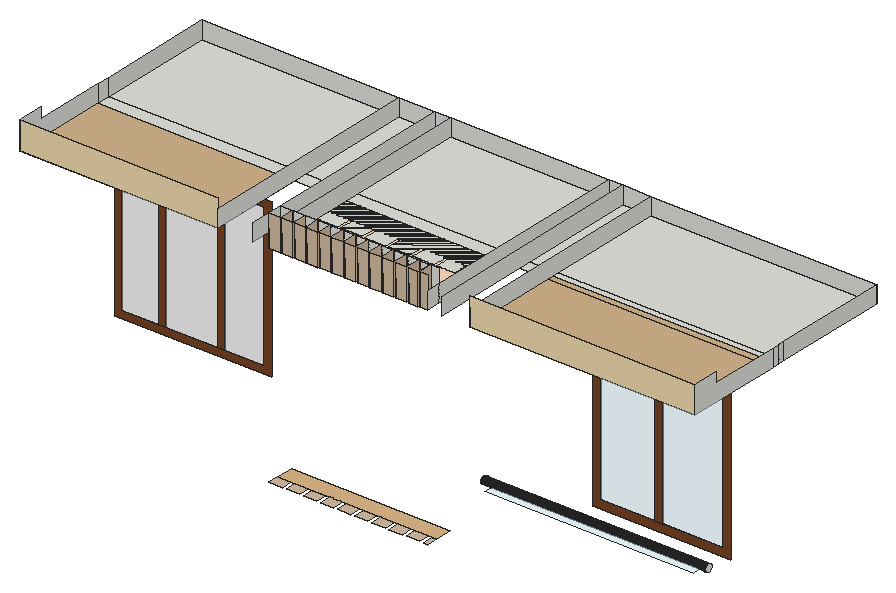
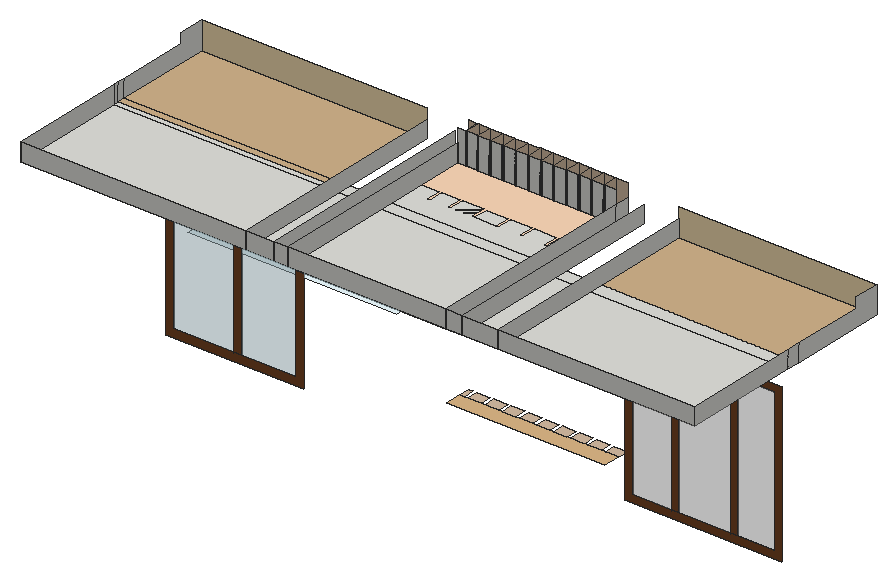
# SketchUp Ruby script. Lengths in inches.
U = 1.inch
M = Sketchup.active_model
def pt(a) = Geom::Point3d.new(a.map { |v| v * U })
def face(e, loops, mat)
  f = e.add_face(loops[0].map { |a| pt(a) })
  loops[1..].each { |l| e.add_face(l.map { |a| pt(a) }).erase! }
  f.material = f.back_material = mat if mat
  f
end
# faces: each face lists its corners as indices into pts; further lists are holes
def faces(e, pts, list, mat = nil) = list.each { |f| face(e, (f[0].is_a?(Array) ? f : [f]).map { |l| l.map { |i| pts[i] } }, mat) }
# xy, xz, yz: faces in a plane at the given z, y or x. An outline is a flat list of corners, or four numbers for a rectangle; further outlines are holes
def ring(l) = l.size == 4 ? [[l[0], l[1]], [l[2], l[1]], [l[2], l[3]], [l[0], l[3]]] : l.each_slice(2).to_a
def flat(e, list, mat, &to3) = list.each { |f| face(e, (f[0].is_a?(Array) ? f : [f]).map { |l| ring(l).map { |u, v| to3.(u, v) } }, mat) }
def xy(e, z, list, mat = nil) = flat(e, list, mat) { |x, y| [x, y, z] }
def xz(e, y, list, mat = nil) = flat(e, list, mat) { |x, z| [x, y, z] }
def yz(e, x, list, mat = nil) = flat(e, list, mat) { |y, z| [x, y, z] }
def lines(e, pts, list) = list.each { |a, b| e.add_line(pt(pts[a]), pt(pts[b])) }
# prism: a flat outline (further loops are holes) pulled along v
def prism(e, loops, v, mat = nil)
  f = face(e, loops, mat); d = Geom::Vector3d.new(v.map { |x| x * U })
  f.pushpull(f.normal.samedirection?(d) ? d.length : -d.length)
end
def box(e, o, s, mat = nil) = prism(e, [[o, [o[0] + s[0], o[1], o[2]], [o[0] + s[0], o[1] + s[1], o[2]], [o[0], o[1] + s[1], o[2]]]], [0, 0, s[2]], mat)
def at(x, y, z, deg = 0) = Geom::Transformation.translation(pt([x, y, z])) * Geom::Transformation.rotation(ORIGIN, Z_AXIS, deg.degrees)
def axes(o, x, y, z) = Geom::Transformation.new([*x, 0, *y, 0, *z, 0, *pt(o).to_a, 1])
def part(name) = M.definitions.add(name)
# library, detail: a bought-in or finely detailed component or shape, given as its bounding box
def library(name, o, s) = part(name).tap { |d| box(d.entities, o, s) }
def detail(e, o, s) = box(e.add_group.entities, o, s)
def put(e, d, t, mat = nil) = e.add_instance(d, t).tap { |i| i.material = mat if mat }
def group(e, t, mat = nil) = e.add_group.tap { |g| g.transformation = t; g.material = mat if mat }.entities
root = M.entities
M.materials.add("[0027_PeachPuff]").color = [255, 218, 185]
M.materials.add("[0034_Wheat]").color = [245, 222, 179]
M.materials.add("[0035_Tan]").color = [210, 180, 140]
M.materials.add("[0036_BurlyWood]1").color = [222, 184, 135]
M.materials.add("[Formica Laminate Dark]").color = [50, 53, 60]
M.materials.add("[Formica Laminate Light]").color = [213, 189, 164]
M.materials.add("[Translucent Glass Gray]").color = [191, 191, 191]
M.materials["[Translucent Glass Gray]"].alpha = 0.5
M.materials.add("[Translucent Glass Safety]").color = [204, 235, 244]
M.materials["[Translucent Glass Safety]"].alpha = 0.5
M.materials.add("[Wood Veneer 01]").color = [120, 70, 37]
xy(root,1718.875,[[800.41,328.44,1272.8,378.54]],"[0036_BurlyWood]1")
xy(root,1718.875,[[800.41,295.82,840.05,328.44],[851.53,295.82,891.17,328.44],[902.66,295.82,942.3,328.44],[953.78,295.82,993.42,328.44],[1004.91,295.82,1044.55,328.44],
  [1056.03,295.82,1095.67,328.44],[1107.16,295.82,1146.8,328.44],[1158.28,295.82,1197.92,328.44],[1209.41,295.82,1249.05,328.44],[1260.53,295.82,1272.8,328.44]],"[Formica Laminate Light]")
xy(root,1901.1875,[[1423.33,322.36,2046.06,378.54]],"[Translucent Glass Safety]")
xy(root,1912.73,[[2056.33,338.97,2057.37,339.03,2058.4,339.19,2059.4,339.47,2060.37,339.85,2061.29,340.33,2062.16,340.9,2062.97,341.56,2063.7,342.3,2064.35,343.11,2064.91,343.98,2065.38,344.91,2065.75,345.89,2066.01,346.89,2066.17,347.92,2066.21,348.96,2066.15,350,2065.98,351.02,2065.71,352.03,2065.33,353,2064.85,353.92,2064.28,354.79,2063.625,355.59,2062.88,356.33,2062.07,356.98,2061.2,357.54,2060.27,358,2059.29,358.37,2058.29,358.64,2057.26,358.79,2056.22,358.84,2055.18,358.78,2054.15,358.61,2053.15,358.34,2052.18,357.96,2051.26,357.48,2050.39,356.91,2049.58,356.25,2048.85,355.51,2048.2,354.7,2047.64,353.82,2047.18,352.89,2046.81,351.92,2046.54,350.91,2046.39,349.89,2046.34,348.85,2046.4,347.81,2046.57,346.78,2046.84,345.78,2047.22,344.81,2047.7,343.89,2048.27,343.02,2048.93,342.21,2049.67,341.48,2050.48,340.83,2051.36,340.27,2052.29,339.8,2053.26,339.43,2054.27,339.17,2055.29,339.01]])
xy(root,1916.77,[[1413.02,338.97,1414.06,339.03,1415.09,339.19,1416.09,339.47,1417.06,339.85,1417.98,340.33,1418.85,340.9,1419.66,341.56,1420.39,342.3,1421.04,343.11,1421.6,343.98,1422.07,344.91,1422.43,345.89,1422.7,346.89,1422.85,347.92,1422.9,348.96,1422.84,350,1422.67,351.02,1422.4,352.03,1422.02,353,1421.54,353.92,1420.97,354.79,1420.3125,355.59,1419.57,356.33,1418.76,356.98,1417.88,357.54,1416.95,358,1415.98,358.37,1414.97,358.64,1413.95,358.79,1412.91,358.84,1411.87,358.78,1410.84,358.61,1409.84,358.34,1408.87,357.96,1407.95,357.48,1407.08,356.91,1406.27,356.25,1405.54,355.51,1404.89,354.7,1404.33,353.82,1403.86,352.89,1403.5,351.92,1403.23,350.91,1403.08,349.89,1403.03,348.85,1403.09,347.81,1403.26,346.78,1403.53,345.78,1403.91,344.81,1404.39,343.89,1404.96,343.02,1405.62,342.21,1406.36,341.48,1407.17,340.83,1408.04,340.27,1408.97,339.8,1409.95,339.43,1410.95,339.17,1411.98,339.01]])
xy(root,2344.3125,[[800.41,474.79,800.41,584.29,1272.8,584.29,1272.8,474.79,1220.42,474.79,1220.42,517.1,1210.375,517.1,1210.375,474.79,1157.91,474.79,1157.91,517.1,1148.92,517.1,1148.92,474.79,1086.41,474.79,1086.41,517.1,1077.42,517.1,1077.42,474.79,1014.91,474.79,1014.91,517.1,1005.92,517.1,1005.92,474.79,943.41,474.79,943.41,517.1,934.42,517.1,934.42,474.79,871.91,474.79,871.91,517.1,862.92,517.1,862.92,474.79],[800.41,474.79,862.92,517.1],[871.91,474.79,934.42,517.1],[943.41,474.79,1005.92,517.1],[1014.91,474.79,1077.42,517.1],
  [1086.41,474.79,1148.92,517.1],[1157.91,474.79,1210.375,517.1],[1220.42,474.79,1272.8,517.1],[800.41,517.1,1272.8,584.29],[58.44,584.29,646.67,623.89],
  [646.67,584.29,752.97,623.89],[752.97,584.29,800.41,623.89],[800.41,584.29,1272.8,623.89],[1272.8,584.29,1313.62,623.89],[1313.62,584.29,1398.32,623.89],
  [1398.32,606.67,2069.85,623.89],[58.44,623.89,646.67,971.67],[646.67,623.89,752.97,971.67],[752.97,623.89,800.41,971.67],[800.41,623.89,1272.8,971.67],
  [1272.8,623.89,1313.62,971.67],[1313.62,623.89,1398.32,971.67],[1398.32,623.89,2069.85,971.67]])
xy(root,2344.3125,[[800.41,339.19,800.41,474.79,862.92,474.79,862.92,517.1,871.91,517.1,871.91,474.79,934.42,474.79,934.42,517.1,943.41,517.1,943.41,474.79,1005.92,474.79,1005.92,517.1,1014.91,517.1,1014.91,474.79,1077.42,474.79,1077.42,517.1,1086.41,517.1,1086.41,474.79,1148.92,474.79,1148.92,517.1,1157.91,517.1,1157.91,474.79,1210.375,474.79,1210.375,517.1,1220.42,517.1,1220.42,474.79,1272.8,474.79,1272.8,339.19]],"[0027_PeachPuff]")
xy(root,2344.3125,[[58.44,295.82,646.67,584.29],[1398.32,295.82,2069.85,584.29],[1398.32,584.29,2069.85,606.67]],"[0035_Tan]")
xy(root,2344.3125,[[800.41,295.82,833.75,339.19],[838.03,295.82,871.37,339.19],[875.66,295.82,909,339.19],[913.28,295.82,946.62,339.19],[950.91,295.82,984.25,339.19],
  [988.53,295.82,1021.87,339.19],[1026.16,295.82,1059.5,339.19],[1063.78,295.82,1097.12,339.19],[1101.41,295.82,1134.75,339.19],[1139.03,295.82,1172.37,339.19],
  [1178.03,295.82,1211.37,339.19],[1215.6,295.82,1244.25,339.19],[1248.93,295.82,1272.8,339.19]],"[Formica Laminate Light]")
xz(root,295.82,[[58.44,2344.3125,646.67,2425.875],[1398.32,2344.3125,2069.85,2425.875]],"[0034_Wheat]")
xz(root,295.82,[[800.41,2344.3125,833.75,2437.75],[838.03,2344.3125,871.37,2437.75],[875.66,2344.3125,909,2437.75],[913.28,2344.3125,946.62,2437.75],[950.91,2344.3125,984.25,2437.75],
  [988.53,2344.3125,1021.87,2437.75],[1026.16,2344.3125,1059.5,2437.75],[1063.78,2344.3125,1097.12,2437.75],[1101.41,2344.3125,1134.75,2437.75],[1139.03,2344.3125,1172.37,2437.75],
  [1178.03,2344.3125,1211.37,2437.75],[1215.6,2344.3125,1244.25,2437.75],[1248.93,2344.3125,1272.8,2437.75]],"[Formica Laminate Light]")
xz(root,339.19,[[800.41,2344.3125,833.75,2437.75],[838.03,2344.3125,871.37,2437.75],[875.66,2344.3125,909,2437.75],[913.28,2344.3125,946.62,2437.75],[950.91,2344.3125,984.25,2437.75],
  [988.53,2344.3125,1021.87,2437.75],[1026.16,2344.3125,1059.5,2437.75],[1063.78,2344.3125,1097.12,2437.75],[1101.41,2344.3125,1134.75,2437.75],[1139.03,2344.3125,1172.37,2437.75],
  [1178.03,2344.3125,1211.37,2437.75],[1215.6,2344.3125,1244.25,2437.75],[1248.93,2344.3125,1272.8,2437.75]])
xz(root,339.19,[[833.75,2344.3125,838.03,2437.75],[871.37,2344.3125,875.66,2437.75],[909,2344.3125,913.28,2437.75],[946.62,2344.3125,950.91,2437.75],[984.25,2344.3125,988.53,2437.75],
  [1021.87,2344.3125,1026.16,2437.75],[1059.5,2344.3125,1063.78,2437.75],[1097.12,2344.3125,1101.41,2437.75],[1134.75,2344.3125,1139.03,2437.75],[1172.37,2344.3125,1178.03,2437.75],
  [1211.37,2344.3125,1215.6,2437.75],[1244.25,2344.3125,1248.93,2437.75]],"[Formica Laminate Dark]")
xz(root,584.29,[[130.1,1815.79,240.86,2240.42],[262.59,1815.79,415.67,2240.42],[437.41,1815.79,554.73,2240.42]],"[Translucent Glass Gray]")
xz(root,584.29,[[[108.51,1794.2,576.32,2262.01],[130.1,1815.79,554.73,2240.42]],[240.86,1815.79,262.59,2240.42],[415.67,1815.79,437.41,2240.42]],"[Wood Veneer 01]")
xz(root,606.67,[[1541.03,1795.22,1700.8,2206.93],[1725.79,1795.22,1902.79,2206.93]],"[Translucent Glass Safety]")
xz(root,606.67,[[[1516.53,1770.73,1927.28,2231.42],[1541.03,1795.22,1902.79,2206.93]],[1700.8,1795.22,1725.79,2206.93]],"[Wood Veneer 01]")
xz(root,971.67,[[58.44,2344.3125,646.67,2395.75],[646.67,2344.3125,752.97,2395.75],[752.97,2344.3125,800.41,2395.75],[800.41,2344.3125,1272.8,2395.75],[1272.8,2344.3125,1313.62,2395.75],
  [1313.62,2344.3125,1398.32,2395.75],[1398.32,2344.3125,2069.85,2395.75]])
yz(root,58.44,[[295.82,2344.3125,295.82,2425.875,373.05,2425.875,373.05,2395.75,584.29,2395.75,584.29,2344.3125],[584.29,2344.3125,623.89,2395.75],[623.89,2344.3125,971.67,2395.75]])
yz(root,646.67,[[295.82,2344.3125,971.67,2395.75]])
yz(root,752.97,[[295.82,2344.3125,971.67,2395.75]])
yz(root,800.41,[[295.82,2344.3125,339.19,2395.75],[339.19,2344.3125,971.67,2395.75]])
yz(root,833.75,[[295.82,2344.3125,339.19,2437.75]],"[Formica Laminate Light]")
yz(root,838.03,[[295.82,2344.3125,339.19,2395.75]],"[Formica Laminate Light]")
yz(root,871.37,[[295.82,2344.3125,339.19,2437.75]],"[Formica Laminate Light]")
yz(root,875.66,[[295.82,2344.3125,339.19,2395.75]],"[Formica Laminate Light]")
yz(root,909,[[295.82,2344.3125,339.19,2437.75]],"[Formica Laminate Light]")
yz(root,913.28,[[295.82,2344.3125,339.19,2395.75]],"[Formica Laminate Light]")
yz(root,946.62,[[295.82,2344.3125,339.19,2437.75]],"[Formica Laminate Light]")
yz(root,950.91,[[295.82,2344.3125,339.19,2395.75]],"[Formica Laminate Light]")
yz(root,984.25,[[295.82,2344.3125,339.19,2437.75]],"[Formica Laminate Light]")
yz(root,988.53,[[295.82,2344.3125,339.19,2395.75]],"[Formica Laminate Light]")
yz(root,1021.87,[[295.82,2344.3125,339.19,2437.75]],"[Formica Laminate Light]")
yz(root,1026.16,[[295.82,2344.3125,339.19,2395.75]],"[Formica Laminate Light]")
yz(root,1059.5,[[295.82,2344.3125,339.19,2437.75]],"[Formica Laminate Light]")
yz(root,1063.78,[[295.82,2344.3125,339.19,2395.75]],"[Formica Laminate Light]")
yz(root,1097.12,[[295.82,2344.3125,339.19,2437.75]],"[Formica Laminate Light]")
yz(root,1101.41,[[295.82,2344.3125,339.19,2395.75]],"[Formica Laminate Light]")
yz(root,1134.75,[[295.82,2344.3125,339.19,2437.75]],"[Formica Laminate Light]")
yz(root,1139.03,[[295.82,2344.3125,339.19,2395.75]],"[Formica Laminate Light]")
yz(root,1172.37,[[295.82,2344.3125,339.19,2437.75]],"[Formica Laminate Light]")
yz(root,1178.03,[[295.82,2344.3125,339.19,2395.75]],"[Formica Laminate Light]")
yz(root,1211.37,[[295.82,2344.3125,339.19,2437.75]],"[Formica Laminate Light]")
yz(root,1215.6,[[295.82,2344.3125,339.19,2395.75]],"[Formica Laminate Light]")
yz(root,1244.25,[[295.82,2344.3125,339.19,2437.75]],"[Formica Laminate Light]")
yz(root,1248.93,[[295.82,2344.3125,339.19,2437.75]],"[Formica Laminate Light]")
yz(root,1272.8,[[295.82,2344.3125,339.19,2395.75],[339.19,2344.3125,971.67,2395.75]])
yz(root,1313.62,[[295.82,2344.3125,971.67,2395.75]])
yz(root,1398.32,[[295.82,2344.3125,971.67,2395.75]])
yz(root,2069.85,[[347.7,1902.74,348.74,1902.79,349.77,1902.95,350.78,1903.21,351.75,1903.58,352.68,1904.04,353.56,1904.6,354.37,1905.25,355.11,1905.99,355.77,1906.79,356.34,1907.66,356.82,1908.58,357.2,1909.55,357.47,1910.56,357.64,1911.58,357.7,1912.62,357.65,1913.66,357.49,1914.6875,357.23,1915.69,356.86,1916.67,356.4,1917.6,355.83,1918.47,355.18,1919.28,354.45,1920.02,353.65,1920.68,352.78,1921.26,351.86,1921.73,350.89,1922.11,349.88,1922.39,348.86,1922.55,347.82,1922.62,346.78,1922.57,345.75,1922.41,344.75,1922.15,343.77,1921.78,342.84,1921.3125,341.97,1920.75,341.15,1920.1,340.41,1919.37,339.76,1918.56,339.18,1917.7,338.71,1916.77,338.33,1915.8,338.05,1914.8,337.88,1913.77,337.82,1912.73,337.87,1911.7,338.03,1910.67,338.29,1909.66,338.66,1908.6875,339.13,1907.76,339.6875,1906.88,340.34,1906.07,341.07,1905.33,341.875,1904.67,342.74,1904.1,343.67,1903.62,344.64,1903.24,345.64,1902.97,346.67,1902.8],[295.82,2344.3125,584.29,2344.3125,584.29,2395.75,373.05,2395.75,373.05,2425.875,295.82,2425.875],[584.29,2344.3125,606.67,2395.75],[606.67,2344.3125,623.89,2395.75],[623.89,2344.3125,971.67,2395.75]])
p = [[2069.85,347.7,1902.74],[2069.85,346.67,1902.8],[1398.32,346.67,1902.8],[1398.32,347.7,1902.74],[2069.85,348.74,1902.79],[1398.32,348.74,1902.79],
  [2069.85,345.64,1902.97],[1398.32,345.64,1902.97],[2069.85,349.77,1902.95],[1398.32,349.77,1902.95],[2069.85,350.78,1903.21],[1398.32,350.78,1903.21],
  [2069.85,344.64,1903.24],[1398.32,344.64,1903.24],[2069.85,343.67,1903.62],[1398.32,343.67,1903.62],[2069.85,351.75,1903.58],[1398.32,351.75,1903.58],
  [2069.85,342.74,1904.1],[1398.32,342.74,1904.1],[2069.85,352.68,1904.04],[1398.32,352.68,1904.04],[2069.85,353.56,1904.6],[1398.32,353.56,1904.6],
  [2069.85,341.875,1904.67],[1398.32,341.875,1904.67],[2069.85,354.37,1905.25],[1398.32,354.37,1905.25],[2069.85,341.07,1905.33],[1398.32,341.07,1905.33],
  [2069.85,340.34,1906.07],[1398.32,340.34,1906.07],[2069.85,355.11,1905.99],[1398.32,355.11,1905.99],[2069.85,355.77,1906.79],[1398.32,355.77,1906.79],
  [2069.85,339.6875,1906.88],[1398.32,339.6875,1906.88],[2069.85,356.34,1907.66],[1398.32,356.34,1907.66],[2069.85,339.13,1907.76],[1398.32,339.13,1907.76],
  [2069.85,356.82,1908.58],[1398.32,356.82,1908.58],[2069.85,338.66,1908.6875],[1398.32,338.66,1908.6875],[2069.85,357.2,1909.55],[1398.32,357.2,1909.55],
  [2069.85,338.29,1909.66],[1398.32,338.29,1909.66],[2069.85,357.47,1910.56],[1398.32,357.47,1910.56],[2069.85,338.03,1910.67],[1398.32,338.03,1910.67],
  [2069.85,357.64,1911.58],[1398.32,357.64,1911.58],[2069.85,337.87,1911.7],[1398.32,337.87,1911.7],[2069.85,357.7,1912.62],[1398.32,357.7,1912.62],
  [2069.85,337.82,1912.73],[1398.32,337.82,1912.73],[2069.85,357.65,1913.66],[1398.32,357.65,1913.66],[2069.85,337.88,1913.77],[1398.32,337.88,1913.77],
  [2069.85,357.49,1914.6875],[1398.32,357.49,1914.6875],[2069.85,338.05,1914.8],[1398.32,338.05,1914.8],[2069.85,357.23,1915.69],[1398.32,357.23,1915.69],
  [2069.85,338.33,1915.8],[1398.32,338.33,1915.8],[2069.85,356.86,1916.67],[1398.32,356.86,1916.67],[2069.85,338.71,1916.77],[1398.32,338.71,1916.77],
  [2069.85,356.4,1917.6],[1398.32,356.4,1917.6],[2069.85,339.18,1917.7],[1398.32,339.18,1917.7],[2069.85,355.83,1918.47],[1398.32,355.83,1918.47],
  [2069.85,339.76,1918.56],[1398.32,339.76,1918.56],[2069.85,355.18,1919.28],[1398.32,355.18,1919.28],[2069.85,340.41,1919.37],[1398.32,340.41,1919.37],
  [2069.85,354.45,1920.02],[1398.32,354.45,1920.02],[2069.85,341.15,1920.1],[1398.32,341.15,1920.1],[2069.85,353.65,1920.68],[1398.32,353.65,1920.68],
  [2069.85,341.97,1920.75],[1398.32,341.97,1920.75],[2069.85,352.78,1921.26],[1398.32,352.78,1921.26],[2069.85,342.84,1921.3125],[1398.32,342.84,1921.3125],
  [2069.85,343.77,1921.78],[1398.32,343.77,1921.78],[2069.85,351.86,1921.73],[1398.32,351.86,1921.73],[2069.85,350.89,1922.11],[1398.32,350.89,1922.11],
  [2069.85,344.75,1922.15],[1398.32,344.75,1922.15],[2069.85,345.75,1922.41],[1398.32,345.75,1922.41],[2069.85,349.88,1922.39],[1398.32,349.88,1922.39],
  [2069.85,346.78,1922.57],[1398.32,346.78,1922.57],[2069.85,348.86,1922.55],[1398.32,348.86,1922.55],[2069.85,347.82,1922.62],[1398.32,347.82,1922.62]]
faces(root,p,[[0,1,2,3],[4,0,3,5],[1,6,7,2],[8,4,5,9],[10,8,9,11],[6,12,13,7],[12,14,15,13],[16,10,11,17],
  [14,18,19,15],[20,16,17,21],[22,20,21,23],[18,24,25,19],[26,22,23,27],[24,28,29,25],[28,30,31,29],[32,26,27,33],
  [34,32,33,35],[30,36,37,31],[38,34,35,39],[36,40,41,37],[42,38,39,43],[40,44,45,41],[46,42,43,47],[44,48,49,45],
  [50,46,47,51],[48,52,53,49],[54,50,51,55],[52,56,57,53],[58,54,55,59],[56,60,61,57],[62,58,59,63],[60,64,65,61],
  [66,62,63,67],[64,68,69,65],[70,66,67,71],[68,72,73,69],[74,70,71,75],[72,76,77,73],[78,74,75,79],[76,80,81,77],
  [82,78,79,83],[80,84,85,81],[86,82,83,87],[84,88,89,85],[90,86,87,91],[88,92,93,89],[94,90,91,95],[92,96,97,93],
  [98,94,95,99],[96,100,101,97],[100,102,103,101],[104,98,99,105],[106,104,105,107],[102,108,109,103],[108,110,111,109],[112,106,107,113],
  [110,114,115,111],[116,112,113,117],[114,118,119,115],[118,116,117,119]],"[Formica Laminate Dark]")
